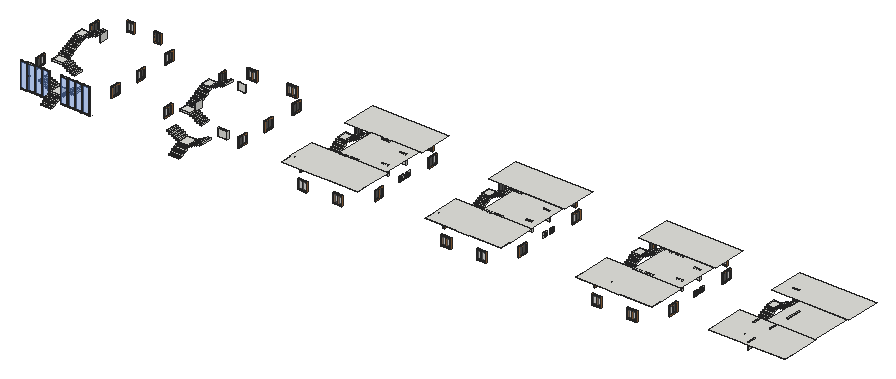
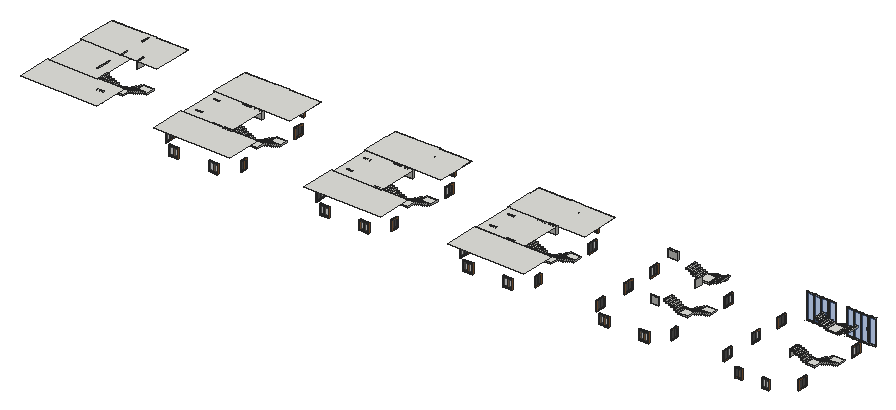
# SketchUp Ruby script. Lengths in inches.
U = 1.inch
M = Sketchup.active_model
def pt(a) = Geom::Point3d.new(a.map { |v| v * U })
def face(e, loops, mat)
  f = e.add_face(loops[0].map { |a| pt(a) })
  loops[1..].each { |l| e.add_face(l.map { |a| pt(a) }).erase! }
  f.material = f.back_material = mat if mat
  f
end
# faces: each face lists its corners as indices into pts; further lists are holes
def faces(e, pts, list, mat = nil) = list.each { |f| face(e, (f[0].is_a?(Array) ? f : [f]).map { |l| l.map { |i| pts[i] } }, mat) }
# xy, xz, yz: faces in a plane at the given z, y or x. An outline is a flat list of corners, or four numbers for a rectangle; further outlines are holes
def ring(l) = l.size == 4 ? [[l[0], l[1]], [l[2], l[1]], [l[2], l[3]], [l[0], l[3]]] : l.each_slice(2).to_a
def flat(e, list, mat, &to3) = list.each { |f| face(e, (f[0].is_a?(Array) ? f : [f]).map { |l| ring(l).map { |u, v| to3.(u, v) } }, mat) }
def xy(e, z, list, mat = nil) = flat(e, list, mat) { |x, y| [x, y, z] }
def xz(e, y, list, mat = nil) = flat(e, list, mat) { |x, z| [x, y, z] }
def yz(e, x, list, mat = nil) = flat(e, list, mat) { |y, z| [x, y, z] }
def lines(e, pts, list) = list.each { |a, b| e.add_line(pt(pts[a]), pt(pts[b])) }
# prism: a flat outline (further loops are holes) pulled along v
def prism(e, loops, v, mat = nil)
  f = face(e, loops, mat); d = Geom::Vector3d.new(v.map { |x| x * U })
  f.pushpull(f.normal.samedirection?(d) ? d.length : -d.length)
end
def box(e, o, s, mat = nil) = prism(e, [[o, [o[0] + s[0], o[1], o[2]], [o[0] + s[0], o[1] + s[1], o[2]], [o[0], o[1] + s[1], o[2]]]], [0, 0, s[2]], mat)
def at(x, y, z, deg = 0) = Geom::Transformation.translation(pt([x, y, z])) * Geom::Transformation.rotation(ORIGIN, Z_AXIS, deg.degrees)
def axes(o, x, y, z) = Geom::Transformation.new([*x, 0, *y, 0, *z, 0, *pt(o).to_a, 1])
def part(name) = M.definitions.add(name)
# library, detail: a bought-in or finely detailed component or shape, given as its bounding box
def library(name, o, s) = part(name).tap { |d| box(d.entities, o, s) }
def detail(e, o, s) = box(e.add_group.entities, o, s)
def put(e, d, t, mat = nil) = e.add_instance(d, t).tap { |i| i.material = mat if mat }
def group(e, t, mat = nil) = e.add_group.tap { |g| g.transformation = t; g.material = mat if mat }.entities
root = M.entities
M.materials.add("[Metal Aluminum Anodized]").color = [202, 209, 219]
M.materials.add("[Translucent Glass Blue]").color = [100, 149, 237]
M.materials["[Translucent Glass Blue]"].alpha = 0.5
M.materials.add("[Translucent Glass Gray]").color = [128, 128, 128]
M.materials["[Translucent Glass Gray]"].alpha = 0.5
M.materials.add("[Translucent_Glass_Gray]").color = [128, 128, 128]
M.materials["[Translucent_Glass_Gray]"].alpha = 0.5
M.materials.add("[Wood Floor]").color = [155, 105, 61]
c1 = part("window")
xy(c1.entities,3.83,[[63.5,0,92.75,0.45],[92.75,0,122,0.23]],"[Metal Aluminum Anodized]")
xy(c1.entities,6,[[8,-0.1,32,0.24],[66,0,90.25,0.45],[95.25,0,119.5,0.23]],"[Metal Aluminum Anodized]")
xy(c1.entities,89.5,[[8,-0.1,32,0.24],[66,0,90.25,0.45],[95.25,0,119.5,0.23]],"[Metal Aluminum Anodized]")
xy(c1.entities,92,[[5.5,-0.1,34.5,0.24],[34.5,0,63.5,0.35],[63.5,0,92.75,0.45],[92.75,0,122,0.23]],"[Metal Aluminum Anodized]")
xz(c1.entities,-0.1,[[8,6,32,89.5]],"[Translucent Glass Blue]")
xz(c1.entities,0,[[63.5,3.5,92.75,3.83],[92.75,3.5,122,3.83]],"[Metal Aluminum Anodized]")
xz(c1.entities,0,[[66,6,90.25,89.5],[95.25,6,119.5,89.5]],"[Translucent Glass Blue]")
xz(c1.entities,0.23,[[[92.75,3.83,122,92],[95.25,6,119.5,89.5]]],"[Metal Aluminum Anodized]")
xz(c1.entities,0.24,[[[5.5,3.83,34.5,92],[8,6,32,89.5]]],"[Metal Aluminum Anodized]")
xz(c1.entities,0.45,[[[63.5,3.83,92.75,92],[66,6,90.25,89.5]]],"[Metal Aluminum Anodized]")
xz(c1.entities,0.45,[[[37,6,61,89.5],[39.25,48.08,39.64,48.15,40.01,48.35,40.32,48.67,40.5625,49.08,40.71,49.57,40.77,50.08,40.71,50.6,40.5625,51.08,40.32,51.5,40.01,51.82,39.64,52.02,39.25,52.08,38.86,52.02,38.49,51.82,38.18,51.5,37.94,51.08,37.79,50.6,37.74,50.08,37.79,49.57,37.94,49.08,38.18,48.67,38.49,48.35,38.86,48.15]]],"[Translucent Glass Blue]")
xz(c1.entities,0.8,[[[34.5,3.83,63.5,92],[37,6,61,89.5]]],"[Metal Aluminum Anodized]")
xz(c1.entities,2.08,[[39.25,48.08,38.86,48.15,38.49,48.35,38.18,48.67,37.94,49.08,37.79,49.57,37.74,50.08,37.79,50.6,37.94,51.08,38.18,51.5,38.49,51.82,38.86,52.02,39.25,52.08,39.64,52.02,40.01,51.82,40.32,51.5,40.5625,51.08,40.71,50.6,40.77,50.08,40.71,49.57,40.5625,49.08,40.32,48.67,40.01,48.35,39.64,48.15]],"[Metal Aluminum Anodized]")
yz(c1.entities,8,[[-0.1,6,0.24,89.5]],"[Metal Aluminum Anodized]")
yz(c1.entities,32,[[-0.1,6,0.24,89.5]],"[Metal Aluminum Anodized]")
yz(c1.entities,34.5,[[0.24,3.83,0.35,92]],"[Metal Aluminum Anodized]")
yz(c1.entities,61,[[0.45,6,0.8,89.5]],"[Metal Aluminum Anodized]")
yz(c1.entities,63.5,[[0.35,3.83,0.45,92]],"[Metal Aluminum Anodized]")
yz(c1.entities,66,[[0,6,0.45,89.5]],"[Metal Aluminum Anodized]")
yz(c1.entities,90.25,[[0,6,0.45,89.5]],"[Metal Aluminum Anodized]")
yz(c1.entities,92.75,[[0.23,3.83,0.45,92]],"[Metal Aluminum Anodized]")
yz(c1.entities,95.25,[[0,6,0.23,89.5]],"[Metal Aluminum Anodized]")
yz(c1.entities,119.5,[[0,6,0.23,89.5]],"[Metal Aluminum Anodized]")
yz(c1.entities,122,[[0,3.83,0.23,92]],"[Metal Aluminum Anodized]")
p = [[39.25,0.45,48.08],[38.86,0.45,48.15],[38.86,2.08,48.15],[39.25,2.08,48.08],[39.64,0.45,48.15],[39.64,2.08,48.15],
  [38.49,0.45,48.35],[38.49,2.08,48.35],[40.01,0.45,48.35],[40.01,2.08,48.35],[38.18,0.45,48.67],[38.18,2.08,48.67],
  [40.32,0.45,48.67],[40.32,2.08,48.67],[37.94,0.45,49.08],[37.94,2.08,49.08],[40.5625,0.45,49.08],[40.5625,2.08,49.08],
  [37.79,0.45,49.57],[37.79,2.08,49.57],[40.71,0.45,49.57],[40.71,2.08,49.57],[37.74,0.45,50.08],[37.74,2.08,50.08],
  [40.77,0.45,50.08],[40.77,2.08,50.08],[37.79,0.45,50.6],[37.79,2.08,50.6],[40.71,0.45,50.6],[40.71,2.08,50.6],
  [37.94,0.45,51.08],[37.94,2.08,51.08],[40.5625,0.45,51.08],[40.5625,2.08,51.08],[38.18,0.45,51.5],[38.18,2.08,51.5],
  [40.32,0.45,51.5],[40.32,2.08,51.5],[38.49,0.45,51.82],[38.49,2.08,51.82],[40.01,0.45,51.82],[40.01,2.08,51.82],
  [38.86,0.45,52.02],[38.86,2.08,52.02],[39.64,0.45,52.02],[39.64,2.08,52.02],[39.25,0.45,52.08],[39.25,2.08,52.08],
  [94.5,0,6],[95.25,0,6],[125.5,0,3.5],[125.5,0,3.83],[125.5,10,3.5],[125.5,10,3.83],
  [34.5,0.35,3.83],[63.5,0.35,3.83],[32,-0.1,6],[33.75,-0.1,6],[34.5,-0.1,3.83],[34.5,0.24,3.83],
  [63.5,0.9,3.83],[63.5,0.9,92]]
faces(c1.entities,p,[[0,1,2,3],[4,0,3,5],[1,6,7,2],[8,4,5,9],[6,10,11,7],[12,8,9,13],[10,14,15,11],[16,12,13,17],
  [14,18,19,15],[20,16,17,21],[18,22,23,19],[24,20,21,25],[22,26,27,23],[28,24,25,29],[26,30,31,27],[32,28,29,33],
  [30,34,35,31],[36,32,33,37],[34,38,39,35],[40,36,37,41],[38,42,43,39],[44,40,41,45],[42,46,47,43],[46,44,45,47]],"[Metal Aluminum Anodized]")
lines(c1.entities,p,[[48,49],[50,51],[52,53],[54,55],[56,57],[58,59],[60,61]])
c2 = part("Group\#105")
box(c2.entities,[0,0,0],[12,46.92,6])
c3 = part("Group\#154")
box(c3.entities,[0,0,0],[12,46.92,6])
c4 = part("Group\#210")
box(c4.entities,[0,0,0],[12,46.92,6])
c5 = part("Group\#267")
box(c5.entities,[0,0,0],[52,12,6])
c6 = part("Group\#339")
box(c6.entities,[0,0,0],[55,12,6])
c7 = part("window full")
xy(c7.entities,0,[[0,0,14.17,66.54]])
xy(c7.entities,2.26,[[12.2,2.26,14.17,64.28]],"[Wood Floor]")
xy(c7.entities,2.36,[[0,2.36,1.97,64.17]],"[Wood Floor]")
xy(c7.entities,3.74,[[11.42,3.74,12.2,32.875],[11.42,33.66,12.2,62.79]],"[Wood Floor]")
xy(c7.entities,3.9375,[[1.97,3.9375,2.76,32.77],[1.97,33.76,2.76,62.6]],"[Wood Floor]")
xy(c7.entities,4.18,[[2.76,4.18,7.09,32.09],[7.09,4.18,11.42,32.09],[2.76,34.45,7.09,62.35],[7.09,34.45,11.42,62.35]],"[Wood Floor]")
xy(c7.entities,69.83,[[2.76,4.18,7.09,32.09],[7.09,32.09,11.42,34.45],[2.76,34.45,7.09,62.35]])
xy(c7.entities,69.83,[[7.09,4.18,11.42,32.09],[7.09,34.45,11.42,62.35]],"[Wood Floor]")
xy(c7.entities,70.08,[[1.97,3.9375,2.76,32.77],[1.97,33.76,2.76,62.6]])
xy(c7.entities,70.27,[[11.42,32.875,12.2,33.66]])
xy(c7.entities,70.27,[[11.42,3.74,12.2,32.875],[11.42,33.66,12.2,62.79]],"[Wood Floor]")
xy(c7.entities,71.65,[[0,2.36,1.97,64.17]])
xy(c7.entities,71.76,[[12.2,2.26,14.17,64.28]],"[Wood Floor]")
xy(c7.entities,74.02,[[0,0,14.17,66.54]],"[Wood Floor]")
xz(c7.entities,0,[[0,0,14.17,74.02]],"[Wood Floor]")
xz(c7.entities,2.26,[[12.2,2.26,14.17,71.76]],"[Wood Floor]")
xz(c7.entities,2.36,[[0,2.36,1.97,71.65]],"[Wood Floor]")
xz(c7.entities,3.74,[[11.42,3.74,12.2,70.27]],"[Wood Floor]")
xz(c7.entities,3.9375,[[1.97,3.9375,2.76,70.08]],"[Wood Floor]")
xz(c7.entities,4.18,[[2.76,4.18,7.09,69.83],[7.09,4.18,11.42,69.83]],"[Wood Floor]")
xz(c7.entities,32.09,[[2.76,4.18,11.42,69.83]],"[Wood Floor]")
xz(c7.entities,32.77,[[1.97,3.9375,2.76,70.08]],"[Wood Floor]")
xz(c7.entities,32.875,[[11.42,3.74,12.2,70.27]],"[Wood Floor]")
xz(c7.entities,33.66,[[11.42,3.74,12.2,47.88],[11.42,47.88,12.2,70.27]],"[Wood Floor]")
xz(c7.entities,33.76,[[1.97,3.9375,2.76,70.08]],"[Wood Floor]")
xz(c7.entities,34.45,[[2.76,4.18,11.42,69.83]],"[Wood Floor]")
xz(c7.entities,62.35,[[2.76,4.18,7.09,69.83],[7.09,4.18,11.42,69.83]],"[Wood Floor]")
xz(c7.entities,62.6,[[1.97,3.9375,2.76,70.08]],"[Wood Floor]")
xz(c7.entities,62.79,[[11.42,3.74,12.2,70.27]],"[Wood Floor]")
xz(c7.entities,64.17,[[0,2.36,1.97,71.65]],"[Wood Floor]")
xz(c7.entities,64.28,[[12.2,2.26,14.17,71.76]],"[Wood Floor]")
xz(c7.entities,66.54,[[0,0,14.17,74.02]],"[Wood Floor]")
yz(c7.entities,0,[[[0,0,66.54,74.02],[2.36,2.36,64.17,71.65]]],"[Wood Floor]")
yz(c7.entities,1.97,[[[2.36,2.36,64.17,71.65],[33.76,3.9375,62.6,70.08],[3.9375,3.9375,32.77,70.08]]],"[Wood Floor]")
yz(c7.entities,2.76,[[32.77,3.9375,33.76,4.18],[32.77,4.18,33.76,69.83],[32.77,69.83,33.76,70.08]])
yz(c7.entities,2.76,[[[3.9375,3.9375,32.77,70.08],[4.18,4.18,32.09,69.83]],[[33.76,3.9375,62.6,70.08],[34.45,4.18,62.35,69.83]]],"[Wood Floor]")
yz(c7.entities,7.09,[[4.18,4.18,62.35,69.83]],"[Translucent Glass Gray]")
yz(c7.entities,11.42,[[32.875,69.83,33.66,70.27]])
yz(c7.entities,11.42,[[[3.74,3.74,32.875,70.27],[4.18,4.18,32.09,69.83]],[[33.66,3.74,62.79,70.27],[34.45,4.18,62.35,69.83]]],"[Wood Floor]")
yz(c7.entities,12.2,[[[2.26,2.26,64.28,71.76],[3.74,3.74,32.875,70.27],[33.66,3.74,62.79,70.27]]],"[Wood Floor]")
yz(c7.entities,14.17,[[[0,0,66.54,74.02],[2.26,2.26,64.28,71.76]]],"[Wood Floor]")
p = [[11.42,32.875,70.27],[11.42,32.875,70.28]]
lines(c7.entities,p,[[0,1]])
c8 = part("Group\#211")
box(c8.entities,[0,0,0],[54,46.92,6])
c9 = part("Group\#268")
box(c9.entities,[0,0,0],[58,59.04,6])
c10 = part("Group\#107")
box(c10.entities,[0,0,0],[46.92,12,6])
c11 = part("Group\#156")
box(c11.entities,[0,0,0],[46.92,12,6])
c12 = part("Group\#212")
box(c12.entities,[0,0,0],[46.92,12,6])
c13 = part("Group\#269")
box(c13.entities,[0,0,0],[12,56.04,6])
c14 = part("Group\#270")
box(c14.entities,[0,0,0],[12,56.04,6])
c15 = part("Group\#343")
p = [[0,43.31,5.11],[2.95,43.31,0],[2.95,0,0],[0,0,5.11]]
faces(c15.entities,p,[[0,1,2,3]],"[Translucent_Glass_Gray]")
c16 = part("Vwntilation+window (1)")
put(c16.entities,c15,at(43.48,1.97,32.29))
put(c16.entities,c15,at(43.48,1.97,26.38))
put(c16.entities,c15,at(43.48,1.97,20.48))
put(c16.entities,c15,at(43.48,1.97,14.57))
put(c16.entities,c15,at(43.48,1.97,8.67))
put(c16.entities,c15,at(43.48,1.97,2.76))
g1 = group(c16.entities,at(43.48,0,0))
prism(g1,[[[1.97,47.24,39.37],[1.97,0,39.37],[1.97,0,0],[1.97,47.24,0]],[[1.97,45.28,1.97],[1.97,1.97,1.97],[1.97,1.97,37.4],[1.97,45.28,37.4]]],[-1.97,0,0])
c17 = part("Group\#219")
box(c17.entities,[0,0,84],[30,4.5,48])
c18 = part("Group\#220")
box(c18.entities,[0,0,84],[30,4.5,48])
c19 = part("Group\#213")
box(c19.entities,[0,0,0],[46.92,46.2,6])
c20 = part("Group\#158")
box(c20.entities,[0,0,0],[12,46.92,6])
c21 = part("Group\#109")
box(c21.entities,[0,0,0],[12,46.92,6])
c22 = part("Group\#214")
box(c22.entities,[0,0,0],[12,46.92,6])
xy(root,132,[[[1499.17,72,1557.17,72,1557.17,75,1718.79,75,1718.79,131.04,1721.79,131.04,1721.79,270,1334.55,270,1334.55,131.04,1337.55,131.04,1337.55,75,1499.17,75],[1343.55,137.04,1476.99,140.04]],[[2226.07,72,2284.07,72,2284.07,75,2445.69,75,2445.69,131.04,2448.69,131.04,2448.69,270,2061.45,270,2061.45,131.04,2064.45,131.04,2064.45,75,2226.07,75],[2070.45,137.04,2203.89,140.04]],[[2988.5,72,3046.5,72,3046.5,75,3208.125,75,3208.125,131.04,3211.125,131.04,3211.125,270,2823.88,270,2823.88,131.04,2826.88,131.04,2826.88,75,2988.5,75],[2832.88,137.04,2966.32,140.04]],[[3661.98,72,3719.98,72,3719.98,75,3881.6,75,3881.6,131.04,3884.6,131.04,3884.6,270,3497.36,270,3497.36,131.04,3500.36,131.04,3500.36,75,3661.98,75],[3506.36,137.04,3639.8,140.04]],[1469.55,270,1712.79,477.12],
  [2196.45,270,2439.69,477.12],[2958.88,270,3202.125,477.12],[3632.36,270,3875.6,477.12],[1334.55,477.12,1721.79,652.56],[2061.45,477.12,2448.69,652.56],
  [2823.88,477.12,3211.125,652.56],[3497.36,477.12,3884.6,652.56]])
p = [[1721.79,72,132],[1721.79,75,132],[1334.55,72,132],[1499.17,72,132],[1557.17,72,132],[1721.79,131.04,132],
  [1334.55,75,132],[1334.55,131.04,132],[2061.45,75,132],[2061.45,72,132],[2061.45,131.04,132],[2284.07,72,132],
  [2448.69,72,132],[2448.69,75,132],[2448.69,131.04,132],[2226.07,72,132],[3046.5,72,132],[3211.125,72,132],
  [2823.88,131.04,132],[2823.88,75,132],[3211.125,75,132],[3211.125,131.04,132],[2823.88,72,132],[2988.5,72,132],
  [3497.36,75,132],[3497.36,72,132],[3884.6,72,132],[3884.6,75,132],[3661.98,72,132],[3719.98,72,132],
  [3497.36,131.04,132],[3884.6,131.04,132]]
lines(root,p,[[0,1],[2,3],[4,0],[1,5],[6,2],[7,6],[8,9],[10,8],[11,12],[13,14],[12,13],[9,15],
  [16,17],[18,19],[20,21],[19,22],[17,20],[22,23],[24,25],[26,27],[25,28],[29,26],[30,24],[27,31]])
put(root,c1,axes([213.75,68.98,-1.71],[1.27,0,0],[0,1,0],[0,0,1.49]))
put(root,c1,axes([10.25,68.98,-1.71],[1.27,0,0],[0,1,0],[0,0,1.49]))
put(root,c2,at(3608.36,279,6))
put(root,c3,at(2934.88,279,6))
put(root,c4,at(2172.45,279,6))
put(root,c5,at(812.93,12,6))
put(root,c6,at(164.62,12,6))
put(root,c4,at(1445.55,279,6))
put(root,c4,at(756.31,279,6))
put(root,c4,at(111,279,6))
put(root,c2,at(3596.36,279,12))
put(root,c3,at(2922.88,279,12))
put(root,c4,at(2160.45,279,12))
put(root,c5,at(812.93,24,12))
put(root,c6,at(164.62,24,12))
put(root,c4,at(1433.55,279,12))
put(root,c4,at(744.31,279,12))
put(root,c4,at(99,279,12))
put(root,c2,at(3584.36,279,18))
put(root,c3,at(2910.88,279,18))
put(root,c4,at(2148.45,279,18))
put(root,c5,at(812.93,36,18))
put(root,c6,at(164.62,36,18))
put(root,c4,at(1421.55,279,18))
put(root,c4,at(732.31,279,18))
put(root,c4,at(87,279,18))
put(root,c2,at(3572.36,279,24))
put(root,c3,at(2898.88,279,24))
put(root,c4,at(2136.45,279,24))
put(root,c5,at(812.93,48,24))
put(root,c6,at(164.62,48,24))
put(root,c4,at(1409.55,279,24))
put(root,c4,at(720.31,279,24))
put(root,c4,at(75,279,24))
put(root,c2,at(3560.36,279,30))
put(root,c3,at(2886.88,279,30))
put(root,c4,at(2124.45,279,30))
put(root,c5,at(812.93,60,30))
put(root,c6,at(164.62,60,30))
put(root,c4,at(1397.55,279,30))
put(root,c4,at(708.31,279,30))
put(root,c4,at(63,279,30))
put(root,c7,axes([704.27,652.93,36],[0,-0.47,0],[0.7145,0,0],[0,0,0.64851]))
put(root,c7,axes([906.19,652.93,36],[0,-0.47,0],[0.7145,0,0],[0,0,0.64851]))
put(root,c7,axes([1595.43,652.93,36],[0,-0.47,0],[0.7145,0,0],[0,0,0.64851]))
put(root,c7,axes([1393.51,652.93,36],[0,-0.47,0],[0.7145,0,0],[0,0,0.64851]))
put(root,c7,axes([2322.33,652.93,36],[0,-0.47,0],[0.7145,0,0],[0,0,0.64851]))
put(root,c7,axes([2120.42,652.93,36],[0,-0.47,0],[0.7145,0,0],[0,0,0.64851]))
put(root,c7,axes([3084.76,652.93,36],[0,-0.47,0],[0.7145,0,0],[0,0,0.64851]))
put(root,c7,axes([2882.85,652.93,36],[0,-0.47,0],[0.7145,0,0],[0,0,0.64851]))
put(root,c7,axes([1595.43,81.37,36],[0,-0.47,0],[0.70736,0,0],[0,0,0.64851]))
put(root,c7,axes([1416.75,81.37,36],[0,-0.47,0],[0.70736,0,0],[0,0,0.64851]))
put(root,c7,axes([2322.33,81.37,36],[0,-0.47,0],[0.70736,0,0],[0,0,0.64851]))
put(root,c7,axes([2143.65,81.37,36],[0,-0.47,0],[0.70736,0,0],[0,0,0.64851]))
put(root,c7,axes([3084.76,81.37,36],[0,-0.47,0],[0.70736,0,0],[0,0,0.64851]))
put(root,c7,axes([2906.08,81.37,36],[0,-0.47,0],[0.70736,0,0],[0,0,0.64851]))
put(root,c7,axes([230.55,652.93,36],[0,-0.47,0],[0.50894,0,0],[0,0,0.64851]))
put(root,c7,axes([94.2,652.93,36],[0,-0.47,0],[0.53565,0,0],[0,0,0.64851]))
put(root,c7,axes([1023.55,530.64,36],[0.47,0,0],[0,0.7124,0],[0,0,0.64851]))
put(root,c7,axes([1023.55,352.92,36],[0.47,0,0],[0,0.7124,0],[0,0,0.64851]))
put(root,c7,axes([2823.88,541.88,36],[0.47,0,0],[0,0.5343,0],[0,0,0.64851]))
put(root,c7,axes([2823.88,190.68,36],[0.47,0,0],[0,0.7124,0],[0,0,0.64851]))
put(root,c7,axes([0,190.68,36],[0.47,0,0],[0,0.7124,0],[0,0,0.64851]))
put(root,c7,axes([0,530.64,36],[0.47,0,0],[0,0.7124,0],[0,0,0.64851]))
put(root,c7,axes([378.24,530.64,36],[0.47,0,0],[0,0.7124,0],[0,0,0.64851]))
put(root,c7,axes([378.24,352.92,36],[0.47,0,0],[0,0.7124,0],[0,0,0.64851]))
put(root,c7,axes([378.24,190.68,36],[0.47,0,0],[0,0.7124,0],[0,0,0.64851]))
put(root,c7,axes([645.31,190.68,36],[0.47,0,0],[0,0.7124,0],[0,0,0.64851]))
put(root,c7,axes([645.31,541.84,36],[0.47,0,0],[0,0.54143,0],[0,0,0.64851]))
put(root,c7,axes([1334.55,541.88,36],[0.47,0,0],[0,0.53986,0],[0,0,0.64851]))
put(root,c7,axes([1334.55,190.68,36],[0.47,0,0],[0,0.7124,0],[0,0,0.64851]))
put(root,c7,axes([1712.79,190.68,36],[0.47,0,0],[0,0.7124,0],[0,0,0.64851]))
put(root,c7,axes([1712.79,530.64,36],[0.47,0,0],[0,0.7124,0],[0,0,0.64851]))
put(root,c7,axes([2061.45,190.68,36],[0.47,0,0],[0,0.7124,0],[0,0,0.64851]))
put(root,c7,axes([2061.45,541.88,36],[0.47,0,0],[0,0.5343,0],[0,0,0.64851]))
put(root,c7,axes([2439.69,190.68,36],[0.47,0,0],[0,0.7124,0],[0,0,0.64851]))
put(root,c7,axes([2439.69,530.64,36],[0.47,0,0],[0,0.7124,0],[0,0,0.64851]))
put(root,c7,axes([3202.125,190.68,36],[0.47,0,0],[0,0.7124,0],[0,0,0.64851]))
put(root,c7,axes([3202.125,530.64,36],[0.47,0,0],[0,0.7124,0],[0,0,0.64851]))
g2 = group(root,at(3506.36,279,36))
box(g2,[0,0,0],[54,46.92,6])
g3 = group(root,at(2832.88,279,36))
box(g3,[0,0,0],[54,46.92,6])
put(root,c8,at(2070.45,279,36))
put(root,c9,at(812.93,72,36))
put(root,c9,at(164.62,72,36))
put(root,c8,at(1343.55,279,36))
put(root,c8,at(654.31,279,36))
put(root,c8,at(9,279,36))
put(root,c7,axes([1023.55,190.68,36],[0.47,0,0],[0,0.7124,0],[0,0,0.64851]))
put(root,c10,at(3513.44,325.92,42))
put(root,c11,at(2832.88,325.92,42))
put(root,c12,at(2070.45,325.92,42))
put(root,c13,at(800.93,75,42))
put(root,c14,at(870.93,75,42))
put(root,c13,at(152.62,75,42))
put(root,c14,at(222.62,75,42))
put(root,c12,at(1343.55,325.92,42))
put(root,c12,at(654.31,325.92,42))
put(root,c12,at(9,325.92,42))
put(root,c10,at(3513.44,337.92,48))
put(root,c11,at(2832.88,337.92,48))
put(root,c12,at(2070.45,337.92,48))
put(root,c13,at(788.93,75,48))
put(root,c14,at(882.93,75,48))
put(root,c13,at(140.62,75,48))
put(root,c14,at(234.62,75,48))
put(root,c12,at(1343.55,337.92,48))
put(root,c12,at(654.31,337.92,48))
put(root,c12,at(9,337.92,48))
put(root,c10,at(3513.44,349.92,54))
put(root,c11,at(2832.88,349.92,54))
put(root,c12,at(2070.45,349.92,54))
put(root,c13,at(776.93,75,54))
put(root,c14,at(894.93,75,54))
put(root,c13,at(128.62,75,54))
put(root,c14,at(246.62,75,54))
put(root,c12,at(1343.55,349.92,54))
put(root,c12,at(654.31,349.92,54))
put(root,c12,at(9,349.92,54))
put(root,c16,axes([2403.24,339.09,60],[1,0,0],[0,0.50715,0],[0,0,0.6096]))
put(root,c16,axes([2403.24,381.7,60],[1,0,0],[0,0.50715,0],[0,0,0.6096]))
put(root,c16,axes([3165.68,339.09,60],[1,0,0],[0,0.50715,0],[0,0,0.6096]))
put(root,c16,axes([3165.68,381.7,60],[1,0,0],[0,0.50715,0],[0,0,0.6096]))
put(root,c10,at(3513.44,361.92,60))
put(root,c11,at(2832.88,361.92,60))
put(root,c12,at(2070.45,361.92,60))
put(root,c13,at(764.93,75,60))
put(root,c14,at(906.93,75,60))
put(root,c13,at(116.62,75,60))
put(root,c14,at(258.62,75,60))
put(root,c12,at(1343.55,361.92,60))
put(root,c12,at(654.31,361.92,60))
put(root,c12,at(9,361.92,60))
put(root,c16,axes([1676.34,381.7,60],[1,0,0],[0,0.50715,0],[0,0,0.6096]))
put(root,c16,axes([1676.34,339.09,60],[1,0,0],[0,0.50715,0],[0,0,0.6096]))
put(root,c10,at(3513.44,373.92,66))
put(root,c11,at(2832.88,373.92,66))
put(root,c12,at(2070.45,373.92,66))
put(root,c13,at(752.93,75,66))
put(root,c14,at(918.93,75,66))
put(root,c13,at(104.62,75,66))
put(root,c14,at(270.62,75,66))
put(root,c12,at(1343.55,373.92,66))
put(root,c12,at(654.31,373.92,66))
put(root,c12,at(9,373.92,66))
put(root,c10,at(3513.44,385.92,72))
put(root,c11,at(2832.88,385.92,72))
put(root,c12,at(2070.45,385.92,72))
put(root,c12,at(1343.55,385.92,72))
put(root,c12,at(654.31,385.92,72))
put(root,c12,at(9,385.92,72))
put(root,c10,at(3513.44,397.92,78))
put(root,c11,at(2832.88,397.92,78))
put(root,c12,at(2070.45,397.92,78))
put(root,c12,at(1343.55,397.92,78))
put(root,c12,at(654.31,397.92,78))
put(root,c12,at(9,397.92,78))
g4 = group(root,at(3550.11,542.56,0))
box(g4,[0,0,84],[30,6,48])
put(root,c10,at(3513.44,409.92,84))
put(root,c11,at(2832.88,409.92,84))
g5 = group(root,at(3142.125,427.62,0))
box(g5,[0,0,84],[30,4.5,48])
g6 = group(root,at(3142.125,315,0))
box(g6,[0,0,84],[30,4.5,48])
put(root,c12,at(2070.45,409.92,84))
put(root,c17,at(2379.69,427.62,0))
put(root,c18,at(2379.69,315,0))
put(root,c12,at(1343.55,409.92,84))
put(root,c12,at(654.31,409.92,84))
put(root,c12,at(9,409.92,84))
put(root,c17,at(1652.79,427.62,0))
put(root,c18,at(1652.79,315,0))
g7 = group(root,at(3513.44,421.92,90))
box(g7,[0,0,0],[46.92,46.24,6])
g8 = group(root,at(2832.88,421.92,90))
box(g8,[0,0,0],[46.92,46.2,6])
put(root,c19,at(2070.45,421.92,90))
put(root,c19,at(1343.55,421.92,90))
put(root,c19,at(654.31,421.92,90))
put(root,c19,at(9,421.92,90))
put(root,c20,at(2879.8,421.2,95.17))
g9 = group(root,at(2196.45,270,0))
box(g9,[0,0,96],[38.88,9,36])
g10 = group(root,at(2958.88,270,0))
box(g10,[0,0,96],[38.88,9,36])
g11 = group(root,at(1469.55,270,0))
box(g11,[0,0,96],[38.88,9,36])
g12 = group(root,at(3680.96,95.04,0))
box(g12,[0,0,96],[4,36,36])
g13 = group(root,at(3598.16,231.12,0))
box(g13,[0,0,96],[4.5,38.88,36])
g14 = group(root,at(3684.74,337.56,0))
box(g14,[0,0,96],[4.5,72,36])
put(root,c21,at(3560.36,421.92,96))
g15 = group(root,at(3015.76,468.12,0))
box(g15,[0,0,96],[39,3,36])
g16 = group(root,at(2958.76,468.12,0))
box(g16,[0,0,96],[39,9,36])
g17 = group(root,at(3015.76,275,0))
box(g17,[0,0,96],[39,4,36])
put(root,c22,at(2117.37,421.2,96))
g18 = group(root,at(2253.33,275,0))
box(g18,[0,0,96],[39,4,36])
g19 = group(root,at(2196.33,468.12,0))
box(g19,[0,0,96],[39,9,36])
g20 = group(root,at(1526.43,275,0))
box(g20,[0,0,96],[39,4,36])
g21 = group(root,at(1526.43,468.12,0))
box(g21,[0,0,96],[39,3,36])
g22 = group(root,at(798.19,468.12,0))
box(g22,[0,0,96],[39,3,36])
g23 = group(root,at(770.33,231.16,0))
box(g23,[0,0,96],[3.98,38.84,36])
g24 = group(root,at(966.55,131.04,0))
box(g24,[0,0,96],[48,9,36])
g25 = group(root,at(132,429.12,0))
box(g25,[0,0,96],[3,39,36])
g26 = group(root,at(3680.97,231.12,0))
box(g26,[0,0,96],[3.99,38.88,35.82])
put(root,c22,at(1390.47,421.2,96))
put(root,c22,at(701.23,421.2,96))
put(root,c22,at(55.92,421.2,96))
put(root,c20,at(2891.8,421.2,101.17))
put(root,c21,at(3572.36,421.92,102))
put(root,c22,at(2129.37,421.2,102))
put(root,c22,at(1402.47,421.2,102))
put(root,c22,at(713.23,421.2,102))
put(root,c22,at(67.92,421.2,102))
put(root,c20,at(2903.8,421.2,107.17))
put(root,c21,at(3584.36,421.92,108))
put(root,c22,at(2141.37,421.2,108))
put(root,c22,at(1414.47,421.2,108))
put(root,c22,at(725.23,421.2,108))
put(root,c22,at(79.92,421.2,108))
put(root,c20,at(2915.8,421.2,113.17))
put(root,c21,at(3596.36,421.92,114))
put(root,c22,at(2153.37,421.2,114))
put(root,c22,at(1426.47,421.2,114))
put(root,c22,at(737.23,421.2,114))
put(root,c22,at(91.92,421.2,114))
put(root,c20,at(2927.8,421.2,119.17))
put(root,c21,at(3608.36,421.92,120))
put(root,c22,at(2165.37,421.2,120))
put(root,c22,at(1438.47,421.2,120))
put(root,c22,at(749.23,421.2,120))
put(root,c22,at(103.92,421.2,120))
put(root,c20,at(2939.8,421.2,125.17))
put(root,c21,at(3620.36,421.92,126))
put(root,c22,at(2177.37,421.2,126))
put(root,c22,at(1450.47,421.2,126))
put(root,c22,at(761.23,421.2,126))
put(root,c22,at(115.92,421.2,126))
